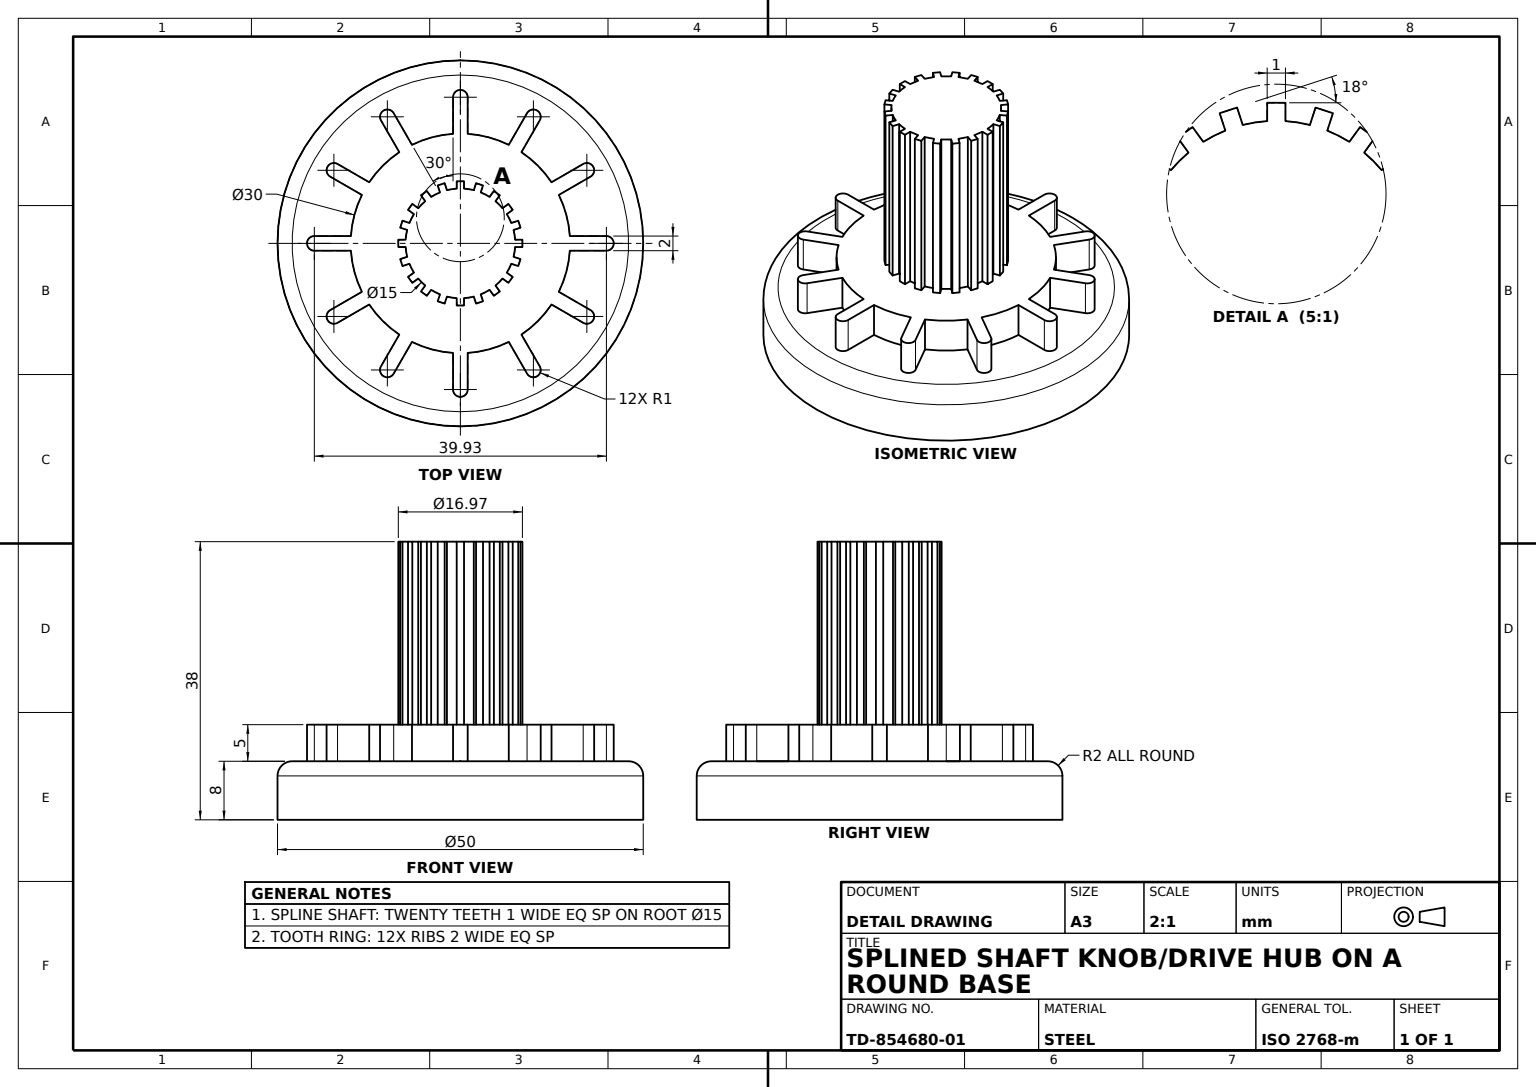
solid
v1 (-0.5,38,-8.483315)
v2 (-0.5,13,-8.483315)
e1 v1 v2 LINE
v3 (0.5,38,-8.483315)
e2 v3 v1 LINE
v4 (0.5,13,-8.483315)
e3 v3 v4 LINE
e4 v4 v2 LINE
face PLANE(AX(P(-0.5,38,-8.483315),D(0,0,1),D(1,0,0))) rev [-e1 -e2 e3 e4]
v5 (-3.097017,38,7.913603)
v6 (-3.097017,13,7.913603)
e5 v5 v6 LINE
v7 (-2.788,38,6.962547)
e6 v7 v5 LINE
v8 (-2.788,13,6.962547)
e7 v7 v8 LINE
e8 v8 v6 LINE
face PLANE(AX(P(-2.788,38,6.962547),D(0.951056516,0,0.309016994),D(0.309016994,0,-0.951056516))) rev [-e5 -e6 e7 e8]
v9 (-4.803091,38,-5.760236)
v10 (-4.803091,13,-5.760236)
e9 v9 v10 LINE
v11 (-5.760236,13,-4.803091)
e10 v10 v11 CIRCLE(AX(P(0,13,0),D(0,1,0),D(0,0,1)),7.5)
v12 (-5.760236,38,-4.803091)
e11 v12 v11 LINE
e12 v9 v12 CIRCLE(AX(P(0,38,0),D(0,1,0),D(0,0,1)),7.5)
face CYL(AX(P(0,38,0),D(0,-1,0),D(0,0,-1)),7.5) [e9 e10 -e11 -e12]
v13 (-7.271564,38,1.836943)
v14 (-7.271564,13,1.836943)
e13 v13 v14 LINE
v15 (-8.22262,13,2.14596)
e14 v14 v15 LINE
v16 (-8.22262,38,2.14596)
e15 v16 v15 LINE
e16 v13 v16 LINE
face PLANE(AX(P(-7.271564,38,1.836943),D(0.309016994,0,0.951056516),D(0.951056516,0,-0.309016994))) rev [e13 e14 -e15 -e16]
v17 (-13.461481,13,-6.617289)
v18 (-13.461481,8,-6.617289)
e17 v17 v18 LINE
v19 (-17.791608,13,-9.117289)
e18 v19 v17 LINE
v20 (-17.791608,8,-9.117289)
e19 v19 v20 LINE
e20 v20 v18 LINE
face PLANE(AX(P(-13.461481,13,-6.617289),D(0.5,0,-0.866025404),D(-0.866025404,0,-0.5))) rev [-e17 -e18 e19 e20]
v21 (-5.760236,13,4.803091)
v22 (-4.803091,13,5.760236)
e21 v21 v22 CIRCLE(AX(P(0,13,0),D(0,1,0),D(0,0,1)),7.5)
v23 (-4.803091,38,5.760236)
e22 v23 v22 LINE
v24 (-5.760236,38,4.803091)
e23 v24 v23 CIRCLE(AX(P(0,38,0),D(0,1,0),D(0,0,1)),7.5)
e24 v24 v21 LINE
face CYL(AX(P(0,38,0),D(0,-1,0),D(0,0,-1)),7.5) [e21 -e22 -e23 e24]
v25 (3.097017,38,-7.913603)
v26 (3.097017,13,-7.913603)
e25 v25 v26 LINE
v27 (2.14596,13,-8.22262)
e26 v26 v27 LINE
v28 (2.14596,38,-8.22262)
e27 v28 v27 LINE
e28 v25 v28 LINE
face PLANE(AX(P(2.14596,38,-8.22262),D(-0.309016994,0,0.951056516),D(0.951056516,0,0.309016994))) rev [e25 e26 -e27 -e28]
v29 (7.157038,38,-4.581859)
v30 (7.157038,13,-4.581859)
e29 v29 v30 LINE
v31 (6.569253,13,-5.390876)
e30 v30 v31 LINE
v32 (6.569253,38,-5.390876)
e31 v32 v31 LINE
e32 v29 v32 LINE
face PLANE(AX(P(6.569253,38,-5.390876),D(-0.809016994,0,0.587785252),D(0.587785252,0,0.809016994))) rev [e29 e30 -e31 -e32]
v33 (7.271564,38,1.836943)
v34 (7.271564,13,1.836943)
e33 v33 v34 LINE
v35 (8.22262,38,2.14596)
e34 v35 v33 LINE
v36 (8.22262,13,2.14596)
e35 v35 v36 LINE
e36 v36 v34 LINE
face PLANE(AX(P(7.271564,38,1.836943),D(-0.309016994,0,0.951056516),D(0.951056516,0,0.309016994))) rev [-e33 -e34 e35 e36]
v37 (-8.483315,38,-0.5)
v38 (-8.483315,38,0.5)
e37 v37 v38 LINE
v39 (-8.483315,13,-0.5)
e38 v37 v39 LINE
v40 (-8.483315,13,0.5)
e39 v39 v40 LINE
e40 v38 v40 LINE
face PLANE(AX(P(-8.483315,38,0.5),D(1,0,0),D(0,0,-1))) rev [-e37 e38 e39 -e40]
v41 (1,8,-14.96663)
v42 (1,8,-19.96663)
e41 v41 v42 LINE
v43 (1,13,-19.96663)
e42 v43 v42 LINE
v44 (1,13,-14.96663)
e43 v44 v43 LINE
e44 v44 v41 LINE
face PLANE(AX(P(1,13,-14.96663),D(-1,0,0),D(0,0,1))) rev [e41 -e42 -e43 e44]
v45 (7.913603,38,3.097017)
e45 v45 v35 LINE
v46 (7.913603,13,3.097017)
e46 v45 v46 LINE
e47 v46 v36 LINE
face PLANE(AX(P(8.22262,38,2.14596),D(-0.951056516,0,-0.309016994),D(-0.309016994,0,0.951056516))) rev [-e45 e46 e47 -e35]
v47 (6.617289,13,13.461481)
v48 (6.617289,8,13.461481)
e48 v47 v48 LINE
v49 (9.117289,8,17.791608)
e49 v48 v49 LINE
v50 (9.117289,13,17.791608)
e50 v50 v49 LINE
e51 v47 v50 LINE
face PLANE(AX(P(6.617289,13,13.461481),D(0.866025404,0,-0.5),D(-0.5,0,-0.866025404))) rev [e48 e49 -e50 -e51]
v51 (-12.461481,13,-8.34934)
v52 (-12.461481,8,-8.34934)
e52 v51 v52 LINE
v53 (-8.34934,13,-12.461481)
e53 v53 v51 CIRCLE(AX(P(0,13,0),D(0,1,0),D(0,0,1)),15)
v54 (-8.34934,8,-12.461481)
e54 v53 v54 LINE
e55 v54 v52 CIRCLE(AX(P(0,8,0),D(0,1,0),D(0,0,1)),15)
face CYL(AX(P(0,13,0),D(0,-1,0),D(0,0,-1)),15) [-e52 -e53 e54 e55]
v55 (5.390876,38,6.569253)
v56 (4.803091,38,5.760236)
e56 v55 v56 LINE
v57 (5.390876,13,6.569253)
e57 v55 v57 LINE
v58 (4.803091,13,5.760236)
e58 v57 v58 LINE
e59 v56 v58 LINE
face PLANE(AX(P(4.803091,38,5.760236),D(-0.809016994,0,0.587785252),D(0.587785252,0,0.809016994))) rev [-e56 e57 e58 -e59]
v59 (7.483315,38,0.5)
e60 v33 v59 CIRCLE(AX(P(0,38,0),D(0,1,0),D(0,0,1)),7.5)
v60 (7.483315,13,0.5)
e61 v34 v60 CIRCLE(AX(P(0,13,0),D(0,1,0),D(0,0,1)),7.5)
e62 v59 v60 LINE
face CYL(AX(P(0,38,0),D(0,-1,0),D(0,0,-1)),7.5) [-e60 e33 e61 -e62]
v61 (3.994074,38,-6.348021)
v62 (3.994074,13,-6.348021)
e63 v61 v62 LINE
v63 (4.581859,38,-7.157038)
e64 v63 v61 LINE
v64 (4.581859,13,-7.157038)
e65 v63 v64 LINE
e66 v64 v62 LINE
face PLANE(AX(P(3.994074,38,-6.348021),D(0.809016994,0,0.587785252),D(0.587785252,0,-0.809016994))) rev [-e63 -e64 e65 e66]
v65 (-7.913603,38,3.097017)
v66 (-6.962547,38,2.788)
e67 v65 v66 LINE
v67 (-7.913603,13,3.097017)
e68 v65 v67 LINE
v68 (-6.962547,13,2.788)
e69 v67 v68 LINE
e70 v66 v68 LINE
face PLANE(AX(P(-6.962547,38,2.788),D(-0.309016994,0,-0.951056516),D(-0.951056516,0,0.309016994))) rev [-e67 e68 e69 -e70]
v69 (1.836943,38,-7.271564)
v70 (1.836943,13,-7.271564)
e71 v69 v70 LINE
e72 v28 v69 LINE
e73 v27 v70 LINE
face PLANE(AX(P(1.836943,38,-7.271564),D(0.951056516,0,0.309016994),D(0.309016994,0,-0.951056516))) rev [-e71 -e72 e27 e73]
v71 (9.117289,8,-17.791608)
v72 (6.617289,8,-13.461481)
e74 v71 v72 LINE
v73 (6.617289,13,-13.461481)
e75 v73 v72 LINE
v74 (9.117289,13,-17.791608)
e76 v74 v73 LINE
e77 v74 v71 LINE
face PLANE(AX(P(6.617289,13,-13.461481),D(0.866025404,0,0.5),D(0.5,0,-0.866025404))) rev [e74 -e75 -e76 e77]
v75 (-1.836943,38,-7.271564)
v76 (-1.836943,13,-7.271564)
e78 v75 v76 LINE
v77 (-2.14596,13,-8.22262)
e79 v76 v77 LINE
v78 (-2.14596,38,-8.22262)
e80 v78 v77 LINE
e81 v75 v78 LINE
face PLANE(AX(P(-1.836943,38,-7.271564),D(-0.951056516,0,0.309016994),D(0.309016994,0,0.951056516))) rev [e78 e79 -e80 -e81]
v79 (-14.96663,8,-1)
e82 v18 v79 CIRCLE(AX(P(0,8,0),D(0,1,0),D(0,0,1)),15)
v80 (-14.96663,13,-1)
e83 v80 v79 LINE
e84 v17 v80 CIRCLE(AX(P(0,13,0),D(0,1,0),D(0,0,1)),15)
face CYL(AX(P(0,13,0),D(0,-1,0),D(0,0,-1)),15) [e17 e82 -e83 -e84]
v81 (1.836943,38,7.271564)
v82 (2.14596,38,8.22262)
e85 v81 v82 LINE
v83 (1.836943,13,7.271564)
e86 v81 v83 LINE
v84 (2.14596,13,8.22262)
e87 v83 v84 LINE
e88 v82 v84 LINE
face PLANE(AX(P(1.836943,38,7.271564),D(0.951056516,0,-0.309016994),D(-0.309016994,0,-0.951056516))) rev [-e85 e86 e87 -e88]
v85 (0,13,-20.96663)
v86 (0,8,-20.96663)
e89 v85 v86 LINE
e90 v43 v85 CIRCLE(AX(P(0,13,-19.96663),D(0,1,0),D(0,0,1)),1)
e91 v42 v86 CIRCLE(AX(P(0,8,-19.96663),D(0,1,0),D(0,0,1)),1)
face CYL(AX(P(0,13,-19.96663),D(0,-1,0),D(0,0,-1)),1) [-e89 -e90 e42 e91]
v87 (13.461481,13,6.617289)
v88 (13.461481,8,6.617289)
e92 v87 v88 LINE
v89 (17.791608,13,9.117289)
e93 v89 v87 LINE
v90 (17.791608,8,9.117289)
e94 v89 v90 LINE
e95 v90 v88 LINE
face PLANE(AX(P(13.461481,13,6.617289),D(-0.5,0,0.866025404),D(0.866025404,0,0.5))) rev [-e92 -e93 e94 e95]
v91 (-0.5,13,8.483315)
v92 (0.5,13,8.483315)
e96 v91 v92 LINE
v93 (0.5,38,8.483315)
e97 v93 v92 LINE
v94 (-0.5,38,8.483315)
e98 v94 v93 LINE
e99 v94 v91 LINE
face PLANE(AX(P(0.5,38,8.483315),D(0,0,-1),D(-1,0,0))) rev [e96 -e97 -e98 e99]
v95 (0.5,38,7.483315)
e100 v95 v81 CIRCLE(AX(P(0,38,0),D(0,1,0),D(0,0,1)),7.5)
v96 (0.5,13,7.483315)
e101 v95 v96 LINE
e102 v96 v83 CIRCLE(AX(P(0,13,0),D(0,1,0),D(0,0,1)),7.5)
face CYL(AX(P(0,38,0),D(0,-1,0),D(0,0,-1)),7.5) [-e100 e101 e102 -e86]
v97 (-8.34934,8,12.461481)
v98 (-10.84934,8,16.791608)
e103 v97 v98 LINE
v99 (-10.84934,13,16.791608)
e104 v99 v98 LINE
v100 (-8.34934,13,12.461481)
e105 v100 v99 LINE
e106 v100 v97 LINE
face PLANE(AX(P(-8.34934,13,12.461481),D(0.866025404,0,0.5),D(0.5,0,-0.866025404))) rev [e103 -e104 -e105 e106]
v101 (5.760236,38,-4.803091)
e107 v32 v101 LINE
v102 (5.760236,13,-4.803091)
e108 v31 v102 LINE
e109 v101 v102 LINE
face PLANE(AX(P(5.760236,38,-4.803091),D(0.587785252,0,0.809016994),D(0.809016994,0,-0.587785252))) rev [-e107 e31 e108 -e109]
v103 (4.581859,38,7.157038)
v104 (4.581859,13,7.157038)
e110 v103 v104 LINE
e111 v104 v57 LINE
e112 v103 v55 LINE
face PLANE(AX(P(5.390876,38,6.569253),D(-0.587785252,0,-0.809016994),D(-0.809016994,0,0.587785252))) rev [e110 e111 -e57 -e112]
v105 (7.271564,38,-1.836943)
v106 (8.22262,38,-2.14596)
e113 v105 v106 LINE
v107 (7.271564,13,-1.836943)
e114 v105 v107 LINE
v108 (8.22262,13,-2.14596)
e115 v107 v108 LINE
e116 v106 v108 LINE
face PLANE(AX(P(7.271564,38,-1.836943),D(-0.309016994,0,-0.951056516),D(-0.951056516,0,0.309016994))) rev [-e113 e114 e115 -e116]
v109 (14.96663,13,-1)
v110 (14.96663,8,-1)
e117 v109 v110 LINE
v111 (19.96663,13,-1)
e118 v111 v109 LINE
v112 (19.96663,8,-1)
e119 v111 v112 LINE
e120 v112 v110 LINE
face PLANE(AX(P(14.96663,13,-1),D(0,0,1),D(1,0,0))) rev [-e117 -e118 e119 e120]
v113 (-9.983315,13,-18.291608)
v114 (-9.983315,8,-18.291608)
e121 v113 v114 LINE
v115 (-9.117289,13,-17.791608)
e122 v115 v113 CIRCLE(AX(P(-9.983315,13,-17.291608),D(0,1,0),D(0,0,1)),1)
v116 (-9.117289,8,-17.791608)
e123 v115 v116 LINE
e124 v116 v114 CIRCLE(AX(P(-9.983315,8,-17.291608),D(0,1,0),D(0,0,1)),1)
face CYL(AX(P(-9.983315,13,-17.291608),D(0,-1,0),D(0,0,-1)),1) [-e121 -e122 e123 e124]
v117 (17.791608,8,-9.117289)
v118 (17.291608,8,-10.983315)
e125 v117 v118 CIRCLE(AX(P(17.291608,8,-9.983315),D(0,1,0),D(0,0,1)),1)
v119 (17.291608,13,-10.983315)
e126 v119 v118 LINE
v120 (17.791608,13,-9.117289)
e127 v120 v119 CIRCLE(AX(P(17.291608,13,-9.983315),D(0,1,0),D(0,0,1)),1)
e128 v120 v117 LINE
face CYL(AX(P(17.291608,13,-9.983315),D(0,-1,0),D(0,0,-1)),1) [e125 -e126 -e127 e128]
v121 (-6.962547,38,-2.788)
v122 (-7.913603,38,-3.097017)
e129 v121 v122 LINE
v123 (-6.962547,13,-2.788)
e130 v121 v123 LINE
v124 (-7.913603,13,-3.097017)
e131 v123 v124 LINE
e132 v122 v124 LINE
face PLANE(AX(P(-6.962547,38,-2.788),D(-0.309016994,0,0.951056516),D(0.951056516,0,0.309016994))) rev [-e129 e130 e131 -e132]
v125 (3.097017,38,7.913603)
v126 (3.097017,13,7.913603)
e133 v125 v126 LINE
v127 (2.788,13,6.962547)
e134 v126 v127 LINE
v128 (2.788,38,6.962547)
e135 v128 v127 LINE
e136 v125 v128 LINE
face PLANE(AX(P(2.788,38,6.962547),D(-0.951056516,0,0.309016994),D(0.309016994,0,0.951056516))) rev [e133 e134 -e135 -e136]
v129 (-5.390876,38,-6.569253)
e137 v129 v9 LINE
v130 (-5.390876,13,-6.569253)
e138 v129 v130 LINE
e139 v130 v10 LINE
face PLANE(AX(P(-4.803091,38,-5.760236),D(0.809016994,0,-0.587785252),D(-0.587785252,0,-0.809016994))) rev [-e137 e138 e139 -e9]
v131 (0,0,25)
v132 (0,0,-25)
e140 v131 v132 CIRCLE(AX(P(0,0,0),D(0,1,0),D(0,0,1)),25)
e141 v132 v131 CIRCLE(AX(P(0,0,0),D(0,1,0),D(0,0,1)),25)
face PLANE(AX(P(0,0,0),D(0,1,0),D(0,0,1))) rev [-e140 -e141]
v133 (-10.84934,13,-16.791608)
v134 (-10.84934,8,-16.791608)
e142 v133 v134 LINE
e143 v134 v54 LINE
e144 v133 v53 LINE
face PLANE(AX(P(-8.34934,13,-12.461481),D(0.866025404,0,-0.5),D(-0.5,0,-0.866025404))) rev [e142 e143 -e54 -e144]
v135 (12.461481,13,8.34934)
v136 (16.791608,13,10.84934)
e145 v135 v136 LINE
v137 (12.461481,8,8.34934)
e146 v135 v137 LINE
v138 (16.791608,8,10.84934)
e147 v137 v138 LINE
e148 v136 v138 LINE
face PLANE(AX(P(12.461481,13,8.34934),D(0.5,0,-0.866025404),D(-0.866025404,0,-0.5))) rev [-e145 e146 e147 -e148]
v139 (-1,13,-19.96663)
e149 v85 v139 CIRCLE(AX(P(0,13,-19.96663),D(0,1,0),D(0,0,1)),1)
v140 (-1,8,-19.96663)
e150 v86 v140 CIRCLE(AX(P(0,8,-19.96663),D(0,1,0),D(0,0,1)),1)
e151 v139 v140 LINE
face CYL(AX(P(0,13,-19.96663),D(0,-1,0),D(0,0,-1)),1) [-e149 e89 e150 -e151]
v141 (-4.581859,38,7.157038)
v142 (-4.581859,13,7.157038)
e152 v141 v142 LINE
v143 (-3.994074,13,6.348021)
e153 v142 v143 LINE
v144 (-3.994074,38,6.348021)
e154 v144 v143 LINE
e155 v141 v144 LINE
face PLANE(AX(P(-3.994074,38,6.348021),D(-0.809016994,0,-0.587785252),D(-0.587785252,0,0.809016994))) rev [e152 e153 -e154 -e155]
v145 (6.962547,38,-2.788)
v146 (6.348021,38,-3.994074)
e156 v145 v146 CIRCLE(AX(P(0,38,0),D(0,1,0),D(0,0,1)),7.5)
v147 (6.962547,13,-2.788)
e157 v145 v147 LINE
v148 (6.348021,13,-3.994074)
e158 v147 v148 CIRCLE(AX(P(0,13,0),D(0,1,0),D(0,0,1)),7.5)
e159 v146 v148 LINE
face CYL(AX(P(0,38,0),D(0,-1,0),D(0,0,-1)),7.5) [-e156 e157 e158 -e159]
e160 v73 v44 CIRCLE(AX(P(0,13,0),D(0,1,0),D(0,0,1)),15)
e161 v72 v41 CIRCLE(AX(P(0,8,0),D(0,1,0),D(0,0,1)),15)
face CYL(AX(P(0,13,0),D(0,-1,0),D(0,0,-1)),15) [-e160 e75 e161 -e44]
v149 (12.461481,8,-8.34934)
v150 (8.34934,8,-12.461481)
e162 v149 v150 CIRCLE(AX(P(0,8,0),D(0,1,0),D(0,0,1)),15)
v151 (8.34934,13,-12.461481)
e163 v151 v150 LINE
v152 (12.461481,13,-8.34934)
e164 v152 v151 CIRCLE(AX(P(0,13,0),D(0,1,0),D(0,0,1)),15)
e165 v152 v149 LINE
face CYL(AX(P(0,13,0),D(0,-1,0),D(0,0,-1)),15) [e162 -e163 -e164 e165]
v153 (19.96663,8,1)
e166 v153 v112 CIRCLE(AX(P(19.96663,8,0),D(0,1,0),D(0,0,1)),1)
v154 (19.96663,13,1)
e167 v154 v111 CIRCLE(AX(P(19.96663,13,0),D(0,1,0),D(0,0,1)),1)
e168 v154 v153 LINE
face CYL(AX(P(19.96663,13,0),D(0,-1,0),D(0,0,-1)),1) [e166 -e119 -e167 e168]
v155 (-1.836943,38,7.271564)
v156 (-1.836943,13,7.271564)
e169 v155 v156 LINE
v157 (-2.14596,38,8.22262)
e170 v157 v155 LINE
v158 (-2.14596,13,8.22262)
e171 v157 v158 LINE
e172 v158 v156 LINE
face PLANE(AX(P(-1.836943,38,7.271564),D(-0.951056516,0,-0.309016994),D(-0.309016994,0,0.951056516))) rev [-e169 -e170 e171 e172]
v159 (3.994074,13,6.348021)
e173 v159 v104 LINE
v160 (3.994074,38,6.348021)
e174 v160 v103 LINE
e175 v160 v159 LINE
face PLANE(AX(P(3.994074,38,6.348021),D(0.809016994,0,-0.587785252),D(-0.587785252,0,-0.809016994))) rev [e173 -e110 -e174 e175]
v161 (-5.390876,38,6.569253)
v162 (-5.390876,13,6.569253)
e176 v161 v162 LINE
e177 v162 v142 LINE
e178 v161 v141 LINE
face PLANE(AX(P(-4.581859,38,7.157038),D(0.587785252,0,-0.809016994),D(-0.809016994,0,-0.587785252))) rev [e176 e177 -e152 -e178]
v163 (13.461481,13,-6.617289)
e179 v163 v120 LINE
v164 (13.461481,8,-6.617289)
e180 v163 v164 LINE
e181 v164 v117 LINE
face PLANE(AX(P(13.461481,13,-6.617289),D(-0.5,0,-0.866025404),D(-0.866025404,0,0.5))) rev [-e179 e180 e181 -e128]
v165 (5.390876,38,-6.569253)
v166 (5.390876,13,-6.569253)
e182 v165 v166 LINE
v167 (4.803091,38,-5.760236)
e183 v167 v165 LINE
v168 (4.803091,13,-5.760236)
e184 v167 v168 LINE
e185 v168 v166 LINE
face PLANE(AX(P(4.803091,38,-5.760236),D(-0.809016994,0,-0.587785252),D(-0.587785252,0,0.809016994))) rev [-e182 -e183 e184 e185]
v169 (0,6,-25)
v170 (0,6,25)
e186 v169 v170 CIRCLE(AX(P(0,6,0),D(0,-1,0),D(0,0,1)),25)
v171 (0,8,-23)
e187 v169 v171 CIRCLE(AX(P(0,6,-23),D(1,0,0),D(0,0,-1)),2)
v172 (0,8,23)
e188 v172 v171 CIRCLE(AX(P(0,8,0),D(0,1,0),D(0,0,1)),23)
e189 v170 v172 CIRCLE(AX(P(0,6,23),D(-1,0,0),D(0,0,1)),2)
face TORUS(AX(P(0,6,0),D(0,1,0),D(0,0,1)),23,2) [-e186 e187 -e188 -e189]
e190 v166 v64 LINE
e191 v165 v63 LINE
face PLANE(AX(P(4.581859,38,-7.157038),D(-0.587785252,0,0.809016994),D(0.809016994,0,0.587785252))) rev [e182 e190 -e65 -e191]
v173 (7.913603,38,-3.097017)
e192 v106 v173 LINE
v174 (7.913603,13,-3.097017)
e193 v108 v174 LINE
e194 v173 v174 LINE
face PLANE(AX(P(7.913603,38,-3.097017),D(-0.951056516,0,0.309016994),D(0.309016994,0,0.951056516))) rev [-e192 e116 e193 -e194]
v175 (14.96663,13,1)
v176 (14.96663,8,1)
e195 v175 v176 LINE
e196 v87 v175 CIRCLE(AX(P(0,13,0),D(0,1,0),D(0,0,1)),15)
e197 v88 v176 CIRCLE(AX(P(0,8,0),D(0,1,0),D(0,0,1)),15)
face CYL(AX(P(0,13,0),D(0,-1,0),D(0,0,-1)),15) [-e195 -e196 e92 e197]
v177 (7.157038,38,4.581859)
v178 (6.348021,38,3.994074)
e198 v177 v178 LINE
v179 (7.157038,13,4.581859)
e199 v177 v179 LINE
v180 (6.348021,13,3.994074)
e200 v179 v180 LINE
e201 v178 v180 LINE
face PLANE(AX(P(6.348021,38,3.994074),D(-0.587785252,0,0.809016994),D(0.809016994,0,0.587785252))) rev [-e198 e199 e200 -e201]
v181 (-19.96663,13,1)
v182 (-14.96663,13,1)
e202 v181 v182 LINE
v183 (-19.96663,8,1)
e203 v181 v183 LINE
v184 (-14.96663,8,1)
e204 v183 v184 LINE
e205 v182 v184 LINE
face PLANE(AX(P(-14.96663,13,1),D(0,0,-1),D(-1,0,0))) rev [-e202 e203 e204 -e205]
v185 (-2.788,38,-6.962547)
v186 (-2.788,13,-6.962547)
e206 v185 v186 LINE
v187 (-3.994074,13,-6.348021)
e207 v186 v187 CIRCLE(AX(P(0,13,0),D(0,1,0),D(0,0,1)),7.5)
v188 (-3.994074,38,-6.348021)
e208 v188 v187 LINE
e209 v185 v188 CIRCLE(AX(P(0,38,0),D(0,1,0),D(0,0,1)),7.5)
face CYL(AX(P(0,38,0),D(0,-1,0),D(0,0,-1)),7.5) [e206 e207 -e208 -e209]
v189 (-13.461481,8,6.617289)
v190 (-17.791608,8,9.117289)
e210 v189 v190 LINE
v191 (-17.791608,13,9.117289)
e211 v191 v190 LINE
v192 (-13.461481,13,6.617289)
e212 v192 v191 LINE
e213 v192 v189 LINE
face PLANE(AX(P(-13.461481,13,6.617289),D(0.5,0,0.866025404),D(0.866025404,0,-0.5))) rev [e210 -e211 -e212 e213]
e214 v127 v159 CIRCLE(AX(P(0,13,0),D(0,1,0),D(0,0,1)),7.5)
e215 v128 v160 CIRCLE(AX(P(0,38,0),D(0,1,0),D(0,0,1)),7.5)
face CYL(AX(P(0,38,0),D(0,-1,0),D(0,0,-1)),7.5) [e135 e214 -e175 -e215]
v193 (-16.791608,8,10.84934)
v194 (-12.461481,8,8.34934)
e216 v193 v194 LINE
v195 (-12.461481,13,8.34934)
e217 v195 v194 LINE
v196 (-16.791608,13,10.84934)
e218 v196 v195 LINE
e219 v196 v193 LINE
face PLANE(AX(P(-12.461481,13,8.34934),D(-0.5,0,-0.866025404),D(-0.866025404,0,0.5))) rev [e216 -e217 -e218 e219]
v197 (-3.097017,38,-7.913603)
e220 v78 v197 LINE
v198 (-3.097017,13,-7.913603)
e221 v77 v198 LINE
e222 v197 v198 LINE
face PLANE(AX(P(-3.097017,38,-7.913603),D(0.309016994,0,0.951056516),D(0.951056516,0,-0.309016994))) rev [-e220 e80 e221 -e222]
v199 (-7.157038,38,-4.581859)
v200 (-7.157038,13,-4.581859)
e223 v199 v200 LINE
v201 (-6.348021,13,-3.994074)
e224 v200 v201 LINE
v202 (-6.348021,38,-3.994074)
e225 v202 v201 LINE
e226 v199 v202 LINE
face PLANE(AX(P(-6.348021,38,-3.994074),D(0.587785252,0,-0.809016994),D(-0.809016994,0,-0.587785252))) rev [e223 e224 -e225 -e226]
e227 v170 v131 LINE
e228 v169 v132 LINE
face CYL(AX(P(0,8,0),D(0,-1,0),D(0,0,-1)),25) [e186 e227 e140 -e228]
v203 (8.483315,38,-0.5)
v204 (7.483315,38,-0.5)
e229 v203 v204 LINE
v205 (8.483315,13,-0.5)
e230 v203 v205 LINE
v206 (7.483315,13,-0.5)
e231 v205 v206 LINE
e232 v204 v206 LINE
face PLANE(AX(P(7.483315,38,-0.5),D(0,0,1),D(1,0,0))) rev [-e229 e230 e231 -e232]
e233 v5 v157 LINE
e234 v6 v158 LINE
face PLANE(AX(P(-2.14596,38,8.22262),D(0.309016994,0,-0.951056516),D(-0.951056516,0,-0.309016994))) rev [-e171 -e233 e5 e234]
e235 v190 v193 CIRCLE(AX(P(-17.291608,8,9.983315),D(0,1,0),D(0,0,1)),1)
e236 v191 v196 CIRCLE(AX(P(-17.291608,13,9.983315),D(0,1,0),D(0,0,1)),1)
face CYL(AX(P(-17.291608,13,9.983315),D(0,-1,0),D(0,0,-1)),1) [e235 -e219 -e236 e211]
e237 v202 v121 CIRCLE(AX(P(0,38,0),D(0,1,0),D(0,0,1)),7.5)
e238 v201 v123 CIRCLE(AX(P(0,13,0),D(0,1,0),D(0,0,1)),7.5)
face CYL(AX(P(0,38,0),D(0,-1,0),D(0,0,-1)),7.5) [-e237 e225 e238 -e130]
v207 (-7.483315,13,0.5)
e239 v40 v207 LINE
v208 (-7.483315,38,0.5)
e240 v208 v207 LINE
e241 v38 v208 LINE
face PLANE(AX(P(-7.483315,38,0.5),D(0,0,-1),D(-1,0,0))) rev [e40 e239 -e240 -e241]
v209 (10.84934,8,-16.791608)
e242 v150 v209 LINE
v210 (10.84934,13,-16.791608)
e243 v210 v209 LINE
e244 v151 v210 LINE
face PLANE(AX(P(8.34934,13,-12.461481),D(-0.866025404,0,-0.5),D(-0.5,0,0.866025404))) rev [e163 e242 -e243 -e244]
v211 (-6.569253,38,5.390876)
v212 (-6.569253,13,5.390876)
e245 v211 v212 LINE
v213 (-7.157038,38,4.581859)
e246 v213 v211 LINE
v214 (-7.157038,13,4.581859)
e247 v213 v214 LINE
e248 v214 v212 LINE
face PLANE(AX(P(-6.569253,38,5.390876),D(0.809016994,0,-0.587785252),D(-0.587785252,0,-0.809016994))) rev [-e245 -e246 e247 e248]
e249 v170 v169 CIRCLE(AX(P(0,6,0),D(0,-1,0),D(0,0,1)),25)
face CYL(AX(P(0,8,0),D(0,-1,0),D(0,0,-1)),25) [e228 e141 -e227 e249]
v215 (2.788,38,-6.962547)
e250 v215 v25 LINE
v216 (2.788,13,-6.962547)
e251 v215 v216 LINE
e252 v216 v26 LINE
face PLANE(AX(P(2.788,38,-6.962547),D(-0.951056516,0,-0.309016994),D(-0.309016994,0,0.951056516))) rev [-e25 -e250 e251 e252]
e253 v136 v89 CIRCLE(AX(P(17.291608,13,9.983315),D(0,1,0),D(0,0,1)),1)
e254 v138 v90 CIRCLE(AX(P(17.291608,8,9.983315),D(0,1,0),D(0,0,1)),1)
face CYL(AX(P(17.291608,13,9.983315),D(0,-1,0),D(0,0,-1)),1) [-e94 -e253 e148 e254]
e255 v101 v167 CIRCLE(AX(P(0,38,0),D(0,1,0),D(0,0,1)),7.5)
e256 v102 v168 CIRCLE(AX(P(0,13,0),D(0,1,0),D(0,0,1)),7.5)
face CYL(AX(P(0,38,0),D(0,-1,0),D(0,0,-1)),7.5) [-e184 -e255 e109 e256]
v217 (-6.348021,38,3.994074)
e257 v66 v217 CIRCLE(AX(P(0,38,0),D(0,1,0),D(0,0,1)),7.5)
v218 (-6.348021,13,3.994074)
e258 v68 v218 CIRCLE(AX(P(0,13,0),D(0,1,0),D(0,0,1)),7.5)
e259 v217 v218 LINE
face CYL(AX(P(0,38,0),D(0,-1,0),D(0,0,-1)),7.5) [-e257 e70 e258 -e259]
v219 (-4.581859,38,-7.157038)
v220 (-4.581859,13,-7.157038)
e260 v219 v220 LINE
e261 v220 v130 LINE
e262 v219 v129 LINE
face PLANE(AX(P(-5.390876,38,-6.569253),D(0.587785252,0,0.809016994),D(0.809016994,0,-0.587785252))) rev [e260 e261 -e138 -e262]
e263 v23 v161 LINE
e264 v22 v162 LINE
face PLANE(AX(P(-4.803091,38,5.760236),D(0.809016994,0,0.587785252),D(0.587785252,0,-0.809016994))) rev [-e176 -e263 e22 e264]
v221 (-0.5,13,7.483315)
e265 v221 v91 LINE
v222 (-0.5,38,7.483315)
e266 v222 v94 LINE
e267 v222 v221 LINE
face PLANE(AX(P(-0.5,38,7.483315),D(1,0,0),D(0,0,-1))) rev [e265 -e99 -e266 e267]
v223 (-1,13,-14.96663)
v224 (-1,8,-14.96663)
e268 v223 v224 LINE
e269 v139 v223 LINE
e270 v140 v224 LINE
face PLANE(AX(P(-1,13,-14.96663),D(1,0,0),D(0,0,-1))) rev [-e268 -e269 e151 e270]
e271 v93 v95 LINE
e272 v92 v96 LINE
face PLANE(AX(P(0.5,38,7.483315),D(-1,0,0),D(0,0,1))) rev [-e101 -e271 e97 e272]
e273 v198 v186 LINE
e274 v197 v185 LINE
face PLANE(AX(P(-2.788,38,-6.962547),D(0.951056516,0,-0.309016994),D(-0.309016994,0,-0.951056516))) rev [e222 e273 -e206 -e274]
v225 (-16.791608,8,-10.84934)
e275 v52 v225 LINE
v226 (-16.791608,13,-10.84934)
e276 v226 v225 LINE
e277 v51 v226 LINE
face PLANE(AX(P(-12.461481,13,-8.34934),D(-0.5,0,0.866025404),D(0.866025404,0,0.5))) rev [e275 -e276 -e277 e52]
v227 (10.84934,13,16.791608)
e278 v50 v227 CIRCLE(AX(P(9.983315,13,17.291608),D(0,1,0),D(0,0,1)),1)
v228 (8.34934,13,12.461481)
e279 v227 v228 LINE
e280 v228 v135 CIRCLE(AX(P(0,13,0),D(0,1,0),D(0,0,1)),15)
e281 v175 v154 LINE
e282 v109 v163 CIRCLE(AX(P(0,13,0),D(0,1,0),D(0,0,1)),15)
v229 (16.791608,13,-10.84934)
e283 v119 v229 CIRCLE(AX(P(17.291608,13,-9.983315),D(0,1,0),D(0,0,1)),1)
e284 v229 v152 LINE
v230 (9.983315,13,-18.291608)
e285 v210 v230 CIRCLE(AX(P(9.983315,13,-17.291608),D(0,1,0),D(0,0,1)),1)
e286 v230 v74 CIRCLE(AX(P(9.983315,13,-17.291608),D(0,1,0),D(0,0,1)),1)
v231 (-6.617289,13,-13.461481)
e287 v223 v231 CIRCLE(AX(P(0,13,0),D(0,1,0),D(0,0,1)),15)
e288 v231 v115 LINE
e289 v113 v133 CIRCLE(AX(P(-9.983315,13,-17.291608),D(0,1,0),D(0,0,1)),1)
v232 (-17.291608,13,-10.983315)
e290 v226 v232 CIRCLE(AX(P(-17.291608,13,-9.983315),D(0,1,0),D(0,0,1)),1)
e291 v232 v19 CIRCLE(AX(P(-17.291608,13,-9.983315),D(0,1,0),D(0,0,1)),1)
v233 (-19.96663,13,-1)
e292 v80 v233 LINE
e293 v233 v181 CIRCLE(AX(P(-19.96663,13,0),D(0,1,0),D(0,0,1)),1)
e294 v182 v192 CIRCLE(AX(P(0,13,0),D(0,1,0),D(0,0,1)),15)
e295 v195 v100 CIRCLE(AX(P(0,13,0),D(0,1,0),D(0,0,1)),15)
v234 (-9.117289,13,17.791608)
e296 v99 v234 CIRCLE(AX(P(-9.983315,13,17.291608),D(0,1,0),D(0,0,1)),1)
v235 (-6.617289,13,13.461481)
e297 v234 v235 LINE
v236 (-1,13,14.96663)
e298 v235 v236 CIRCLE(AX(P(0,13,0),D(0,1,0),D(0,0,1)),15)
v237 (-1,13,19.96663)
e299 v236 v237 LINE
v238 (1,13,19.96663)
e300 v237 v238 CIRCLE(AX(P(0,13,19.96663),D(0,1,0),D(0,0,1)),1)
v239 (1,13,14.96663)
e301 v238 v239 LINE
e302 v239 v47 CIRCLE(AX(P(0,13,0),D(0,1,0),D(0,0,1)),15)
e303 v148 v30 LINE
e304 v174 v147 LINE
e305 v206 v107 CIRCLE(AX(P(0,13,0),D(0,1,0),D(0,0,1)),7.5)
v240 (8.483315,13,0.5)
e306 v240 v205 LINE
e307 v60 v240 LINE
v241 (6.962547,13,2.788)
e308 v241 v46 LINE
e309 v180 v241 CIRCLE(AX(P(0,13,0),D(0,1,0),D(0,0,1)),7.5)
v242 (6.569253,13,5.390876)
e310 v242 v179 LINE
v243 (5.760236,13,4.803091)
e311 v243 v242 LINE
e312 v58 v243 CIRCLE(AX(P(0,13,0),D(0,1,0),D(0,0,1)),7.5)
e313 v84 v126 LINE
e314 v156 v221 CIRCLE(AX(P(0,13,0),D(0,1,0),D(0,0,1)),7.5)
e315 v143 v8 CIRCLE(AX(P(0,13,0),D(0,1,0),D(0,0,1)),7.5)
e316 v212 v21 LINE
e317 v218 v214 LINE
e318 v15 v67 LINE
e319 v207 v14 CIRCLE(AX(P(0,13,0),D(0,1,0),D(0,0,1)),7.5)
v244 (-7.483315,13,-0.5)
e320 v244 v39 LINE
v245 (-7.271564,13,-1.836943)
e321 v245 v244 CIRCLE(AX(P(0,13,0),D(0,1,0),D(0,0,1)),7.5)
v246 (-8.22262,13,-2.14596)
e322 v246 v245 LINE
e323 v124 v246 LINE
v247 (-6.569253,13,-5.390876)
e324 v247 v200 LINE
e325 v11 v247 LINE
e326 v187 v220 LINE
v248 (-0.5,13,-7.483315)
e327 v248 v76 CIRCLE(AX(P(0,13,0),D(0,1,0),D(0,0,1)),7.5)
e328 v2 v248 LINE
v249 (0.5,13,-7.483315)
e329 v249 v4 LINE
e330 v70 v249 CIRCLE(AX(P(0,13,0),D(0,1,0),D(0,0,1)),7.5)
e331 v62 v216 CIRCLE(AX(P(0,13,0),D(0,1,0),D(0,0,1)),7.5)
face PLANE(AX(P(0,13,-19.96663),D(0,1,0),D(0,0,1))) [e278 e279 e280 e145 e253 e93 e196 e281 e167 e118 e282 e179 e127 e283 e284 e164 e244 e285 e286 e76 e160 e43 e90 e149 e269 e287 e288 e122 e289 e144 e53 e277 e290 e291 e18 e84 e292 e293 e202 e294 e212 e236 e218 e295 e105 e296 e297 e298 e299 e300 e301 e302 e51] [-e185 -e256 -e108 -e30 -e303 -e158 -e304 -e193 -e115 -e305 -e231 -e306 -e307 -e61 -e36 -e47 -e308 -e309 -e200 -e310 -e311 -e312 -e58 -e111 -e173 -e214 -e134 -e313 -e87 -e102 -e272 -e96 -e265 -e314 -e172 -e234 -e8 -e315 -e153 -e177 -e264 -e21 -e316 -e248 -e317 -e258 -e69 -e318 -e14 -e319 -e239 -e39 -e320 -e321 -e322 -e323 -e131 -e238 -e224 -e324 -e325 -e10 -e139 -e261 -e326 -e207 -e273 -e221 -e79 -e327 -e328 -e4 -e329 -e330 -e73 -e26 -e252 -e331 -e66 -e190]
e332 v176 v153 LINE
face PLANE(AX(P(14.96663,13,1),D(0,0,-1),D(-1,0,0))) rev [-e281 e195 e332 -e168]
e333 v208 v13 CIRCLE(AX(P(0,38,0),D(0,1,0),D(0,0,1)),7.5)
face CYL(AX(P(0,38,0),D(0,-1,0),D(0,0,-1)),7.5) [-e13 -e333 e240 e319]
v250 (9.983315,8,-18.291608)
e334 v209 v250 CIRCLE(AX(P(9.983315,8,-17.291608),D(0,1,0),D(0,0,1)),1)
e335 v230 v250 LINE
face CYL(AX(P(9.983315,13,-17.291608),D(0,-1,0),D(0,0,-1)),1) [e334 -e335 -e285 e243]
v251 (5.760236,38,4.803091)
e336 v251 v243 LINE
e337 v56 v251 CIRCLE(AX(P(0,38,0),D(0,1,0),D(0,0,1)),7.5)
face CYL(AX(P(0,38,0),D(0,-1,0),D(0,0,-1)),7.5) [-e336 -e337 e59 e312]
v252 (-7.271564,38,-1.836943)
v253 (-7.483315,38,-0.5)
e338 v252 v253 CIRCLE(AX(P(0,38,0),D(0,1,0),D(0,0,1)),7.5)
e339 v252 v245 LINE
e340 v253 v244 LINE
face CYL(AX(P(0,38,0),D(0,-1,0),D(0,0,-1)),7.5) [-e338 e339 e321 -e340]
e341 v171 v172 CIRCLE(AX(P(0,8,0),D(0,1,0),D(0,0,1)),23)
face TORUS(AX(P(0,6,0),D(0,1,0),D(0,0,1)),23,2) [-e341 -e187 -e249 e189]
e342 v253 v37 LINE
face PLANE(AX(P(-7.483315,38,-0.5),D(0,0,1),D(1,0,0))) rev [-e342 e340 e320 -e38]
e343 v144 v7 CIRCLE(AX(P(0,38,0),D(0,1,0),D(0,0,1)),7.5)
face CYL(AX(P(0,38,0),D(0,-1,0),D(0,0,-1)),7.5) [e315 -e7 -e343 e154]
v254 (6.569253,38,5.390876)
e344 v254 v177 LINE
e345 v254 v242 LINE
face PLANE(AX(P(7.157038,38,4.581859),D(-0.809016994,0,-0.587785252),D(-0.587785252,0,0.809016994))) rev [e310 -e199 -e344 e345]
e346 v250 v71 CIRCLE(AX(P(9.983315,8,-17.291608),D(0,1,0),D(0,0,1)),1)
face CYL(AX(P(9.983315,13,-17.291608),D(0,-1,0),D(0,0,-1)),1) [e335 e346 -e77 -e286]
v255 (-0.5,38,-7.483315)
e347 v255 v75 CIRCLE(AX(P(0,38,0),D(0,1,0),D(0,0,1)),7.5)
e348 v255 v248 LINE
face CYL(AX(P(0,38,0),D(0,-1,0),D(0,0,-1)),7.5) [-e78 -e347 e348 e327]
v256 (10.84934,8,16.791608)
e349 v227 v256 LINE
e350 v49 v256 CIRCLE(AX(P(9.983315,8,17.291608),D(0,1,0),D(0,0,1)),1)
face CYL(AX(P(9.983315,13,17.291608),D(0,-1,0),D(0,0,-1)),1) [-e349 -e278 e50 e350]
v257 (16.791608,8,-10.84934)
e351 v229 v257 LINE
e352 v257 v149 LINE
face PLANE(AX(P(12.461481,13,-8.34934),D(0.5,0,0.866025404),D(0.866025404,0,-0.5))) rev [-e284 e351 e352 -e165]
e353 v211 v24 LINE
face PLANE(AX(P(-5.760236,38,4.803091),D(-0.587785252,0,-0.809016994),D(-0.809016994,0,0.587785252))) rev [-e353 e245 e316 -e24]
v258 (-6.617289,8,13.461481)
e354 v235 v258 LINE
v259 (-1,8,14.96663)
e355 v258 v259 CIRCLE(AX(P(0,8,0),D(0,1,0),D(0,0,1)),15)
e356 v236 v259 LINE
face CYL(AX(P(0,13,0),D(0,-1,0),D(0,0,-1)),15) [-e298 e354 e355 -e356]
e357 v114 v134 CIRCLE(AX(P(-9.983315,8,-17.291608),D(0,1,0),D(0,0,1)),1)
face CYL(AX(P(-9.983315,13,-17.291608),D(0,-1,0),D(0,0,-1)),1) [e121 e357 -e142 -e289]
v260 (-17.291608,8,-10.983315)
e358 v260 v20 CIRCLE(AX(P(-17.291608,8,-9.983315),D(0,1,0),D(0,0,1)),1)
e359 v232 v260 LINE
face CYL(AX(P(-17.291608,13,-9.983315),D(0,-1,0),D(0,0,-1)),1) [e358 -e19 -e291 e359]
e360 v225 v260 CIRCLE(AX(P(-17.291608,8,-9.983315),D(0,1,0),D(0,0,1)),1)
face CYL(AX(P(-17.291608,13,-9.983315),D(0,-1,0),D(0,0,-1)),1) [e276 e360 -e359 -e290]
v261 (1,8,19.96663)
e361 v238 v261 LINE
v262 (-1,8,19.96663)
e362 v237 v262 LINE
e363 v262 v261 CIRCLE(AX(P(0,8,19.96663),D(0,1,0),D(0,0,1)),1)
face CYL(AX(P(0,13,19.96663),D(0,-1,0),D(0,0,-1)),1) [-e361 -e300 e362 e363]
e364 v61 v215 CIRCLE(AX(P(0,38,0),D(0,1,0),D(0,0,1)),7.5)
face CYL(AX(P(0,38,0),D(0,-1,0),D(0,0,-1)),7.5) [e331 -e251 -e364 e63]
v263 (6.962547,38,2.788)
e365 v263 v45 LINE
e366 v263 v241 LINE
face PLANE(AX(P(6.962547,38,2.788),D(0.309016994,0,-0.951056516),D(-0.951056516,0,-0.309016994))) rev [-e46 -e365 e366 e308]
v264 (-9.117289,8,17.791608)
e367 v264 v258 LINE
e368 v234 v264 LINE
face PLANE(AX(P(-6.617289,13,13.461481),D(-0.866025404,0,-0.5),D(-0.5,0,0.866025404))) rev [e367 -e354 -e297 e368]
e369 v82 v125 LINE
face PLANE(AX(P(3.097017,38,7.913603),D(-0.309016994,0,-0.951056516),D(-0.951056516,0,0.309016994))) rev [e313 -e133 -e369 e88]
e370 v118 v257 CIRCLE(AX(P(17.291608,8,-9.983315),D(0,1,0),D(0,0,1)),1)
face CYL(AX(P(17.291608,13,-9.983315),D(0,-1,0),D(0,0,-1)),1) [e370 -e351 -e283 e126]
v265 (-6.617289,8,-13.461481)
e371 v231 v265 LINE
e372 v224 v265 CIRCLE(AX(P(0,8,0),D(0,1,0),D(0,0,1)),15)
face CYL(AX(P(0,13,0),D(0,-1,0),D(0,0,-1)),15) [-e371 -e287 e268 e372]
v266 (-8.22262,38,-2.14596)
e373 v266 v246 LINE
e374 v266 v252 LINE
face PLANE(AX(P(-7.271564,38,-1.836943),D(0.309016994,0,-0.951056516),D(-0.951056516,0,-0.309016994))) rev [e373 e322 -e339 -e374]
e375 v188 v219 LINE
face PLANE(AX(P(-3.994074,38,-6.348021),D(-0.809016994,0,0.587785252),D(0.587785252,0,0.809016994))) rev [-e375 e208 e326 -e260]
v267 (0.5,38,-7.483315)
e376 v267 v3 LINE
e377 v267 v249 LINE
face PLANE(AX(P(0.5,38,-7.483315),D(-1,0,0),D(0,0,1))) rev [-e3 -e376 e377 e329]
v268 (8.483315,38,0.5)
e378 v59 v268 LINE
e379 v268 v240 LINE
face PLANE(AX(P(7.483315,38,0.5),D(0,0,-1),D(-1,0,0))) rev [-e378 e62 e307 -e379]
e380 v194 v97 CIRCLE(AX(P(0,8,0),D(0,1,0),D(0,0,1)),15)
face CYL(AX(P(0,13,0),D(0,-1,0),D(0,0,-1)),15) [e217 e380 -e106 -e295]
e381 v155 v222 CIRCLE(AX(P(0,38,0),D(0,1,0),D(0,0,1)),7.5)
face CYL(AX(P(0,38,0),D(0,-1,0),D(0,0,-1)),7.5) [e169 e314 -e267 -e381]
v269 (8.34934,8,12.461481)
e382 v256 v269 LINE
e383 v228 v269 LINE
face PLANE(AX(P(8.34934,13,12.461481),D(-0.866025404,0,0.5),D(0.5,0,0.866025404))) rev [e382 -e383 -e279 e349]
e384 v173 v145 LINE
face PLANE(AX(P(6.962547,38,-2.788),D(0.309016994,0,0.951056516),D(0.951056516,0,-0.309016994))) rev [e304 -e157 -e384 e194]
e385 v265 v116 LINE
face PLANE(AX(P(-6.617289,13,-13.461481),D(-0.866025404,0,0.5),D(0.5,0,0.866025404))) rev [e385 -e123 -e288 e371]
v270 (-19.96663,8,-1)
e386 v79 v270 LINE
e387 v233 v270 LINE
face PLANE(AX(P(-14.96663,13,-1),D(0,0,1),D(1,0,0))) rev [e386 -e387 -e292 e83]
e388 v269 v137 CIRCLE(AX(P(0,8,0),D(0,1,0),D(0,0,1)),15)
v271 (1,8,14.96663)
e389 v271 v48 CIRCLE(AX(P(0,8,0),D(0,1,0),D(0,0,1)),15)
e390 v261 v271 LINE
e391 v259 v262 LINE
e392 v98 v264 CIRCLE(AX(P(-9.983315,8,17.291608),D(0,1,0),D(0,0,1)),1)
e393 v184 v189 CIRCLE(AX(P(0,8,0),D(0,1,0),D(0,0,1)),15)
e394 v270 v183 CIRCLE(AX(P(-19.96663,8,0),D(0,1,0),D(0,0,1)),1)
e395 v110 v164 CIRCLE(AX(P(0,8,0),D(0,1,0),D(0,0,1)),15)
face PLANE(AX(P(0,8,0),D(0,1,0),D(0,0,1))) [-e388 -e382 -e350 -e49 -e389 -e390 -e363 -e391 -e355 -e367 -e392 -e103 -e380 -e216 -e235 -e210 -e393 -e204 -e394 -e386 -e82 -e20 -e358 -e360 -e275 -e55 -e143 -e357 -e124 -e385 -e372 -e270 -e150 -e91 -e41 -e161 -e74 -e346 -e334 -e242 -e162 -e352 -e370 -e125 -e181 -e395 -e120 -e166 -e332 -e197 -e95 -e254 -e147] [e188 e341]
v272 (-6.569253,38,-5.390876)
e396 v272 v247 LINE
e397 v12 v272 LINE
face PLANE(AX(P(-5.760236,38,-4.803091),D(-0.587785252,0,0.809016994),D(0.809016994,0,0.587785252))) rev [e11 e325 -e396 -e397]
e398 v178 v263 CIRCLE(AX(P(0,38,0),D(0,1,0),D(0,0,1)),7.5)
face CYL(AX(P(0,38,0),D(0,-1,0),D(0,0,-1)),7.5) [-e398 e201 e309 -e366]
face CYL(AX(P(-9.983315,13,17.291608),D(0,-1,0),D(0,0,-1)),1) [e392 -e368 -e296 e104]
e399 v16 v65 LINE
face PLANE(AX(P(-7.913603,38,3.097017),D(0.951056516,0,-0.309016994),D(-0.309016994,0,-0.951056516))) rev [-e68 -e399 e15 e318]
e400 v204 v105 CIRCLE(AX(P(0,38,0),D(0,1,0),D(0,0,1)),7.5)
face CYL(AX(P(0,38,0),D(0,-1,0),D(0,0,-1)),7.5) [e305 -e114 -e400 e232]
e401 v251 v254 LINE
face PLANE(AX(P(5.760236,38,4.803091),D(0.587785252,0,-0.809016994),D(-0.809016994,0,-0.587785252))) rev [e336 e311 -e345 -e401]
e402 v239 v271 LINE
face CYL(AX(P(0,13,0),D(0,-1,0),D(0,0,-1)),15) [e389 -e48 -e302 e402]
face CYL(AX(P(-19.96663,13,0),D(0,-1,0),D(0,0,-1)),1) [-e203 -e293 e387 e394]
face CYL(AX(P(0,13,0),D(0,-1,0),D(0,0,-1)),15) [-e180 -e282 e117 e395]
e403 v268 v203 LINE
face PLANE(AX(P(8.483315,38,-0.5),D(-1,0,0),D(0,0,1))) rev [e379 e306 -e230 -e403]
face CYL(AX(P(0,13,0),D(0,-1,0),D(0,0,-1)),15) [e205 e393 -e213 -e294]
e404 v217 v213 LINE
face PLANE(AX(P(-6.348021,38,3.994074),D(0.587785252,0,0.809016994),D(0.809016994,0,-0.587785252))) rev [e259 e317 -e247 -e404]
face PLANE(AX(P(1,13,14.96663),D(-1,0,0),D(0,0,1))) rev [e361 e390 -e402 -e301]
e405 v272 v199 LINE
face PLANE(AX(P(-7.157038,38,-4.581859),D(0.809016994,0,0.587785252),D(0.587785252,0,-0.809016994))) rev [e324 -e223 -e405 e396]
face CYL(AX(P(0,13,0),D(0,-1,0),D(0,0,-1)),15) [e383 e388 -e146 -e280]
e406 v146 v29 LINE
face PLANE(AX(P(6.348021,38,-3.994074),D(-0.587785252,0,-0.809016994),D(-0.809016994,0,0.587785252))) rev [e159 e303 -e29 -e406]
e407 v1 v255 LINE
face PLANE(AX(P(-0.5,38,-7.483315),D(1,0,0),D(0,0,-1))) rev [-e407 e1 e328 -e348]
e408 v122 v266 LINE
face PLANE(AX(P(-8.22262,38,-2.14596),D(0.951056516,0,0.309016994),D(0.309016994,0,-0.951056516))) rev [e323 -e373 -e408 e132]
e409 v69 v267 CIRCLE(AX(P(0,38,0),D(0,1,0),D(0,0,1)),7.5)
face PLANE(AX(P(0,38,0),D(0,1,0),D(0,0,1))) [e333 e16 e399 e67 e257 e404 e246 e353 e23 e263 e178 e155 e343 e6 e233 e170 e381 e266 e98 e271 e100 e85 e369 e136 e215 e174 e112 e56 e337 e401 e344 e198 e398 e365 e45 e34 e60 e378 e403 e229 e400 e113 e192 e384 e156 e406 e32 e107 e255 e183 e191 e64 e364 e250 e28 e72 e409 e376 e2 e407 e347 e81 e220 e274 e209 e375 e262 e137 e12 e397 e405 e226 e237 e129 e408 e374 e338 e342 e37 e241]
face PLANE(AX(P(-1,13,14.96663),D(1,0,0),D(0,0,-1))) rev [-e299 e356 e391 -e362]
face CYL(AX(P(0,38,0),D(0,-1,0),D(0,0,-1)),7.5) [-e409 e71 e330 -e377]
